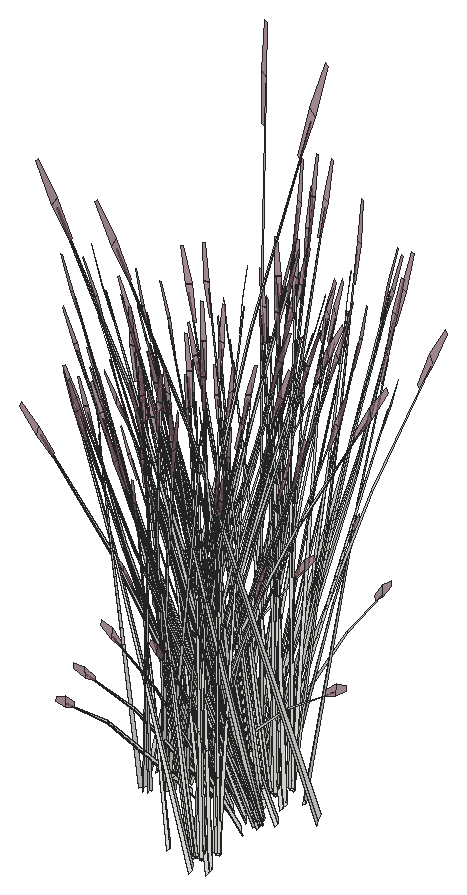
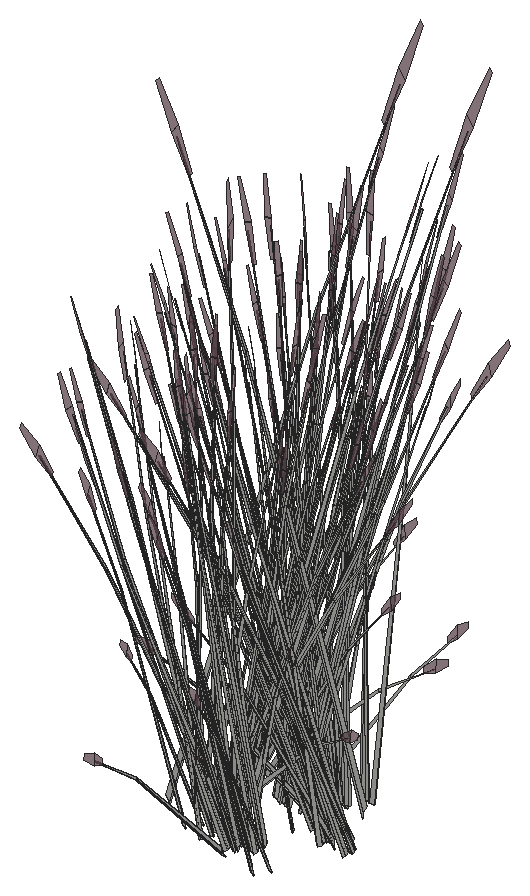
# SketchUp Ruby script. Lengths in inches.
U = 1.inch
M = Sketchup.active_model
def pt(a) = Geom::Point3d.new(a.map { |v| v * U })
def face(e, loops, mat)
  f = e.add_face(loops[0].map { |a| pt(a) })
  loops[1..].each { |l| e.add_face(l.map { |a| pt(a) }).erase! }
  f.material = f.back_material = mat if mat
  f
end
# faces: each face lists its corners as indices into pts; further lists are holes
def faces(e, pts, list, mat = nil) = list.each { |f| face(e, (f[0].is_a?(Array) ? f : [f]).map { |l| l.map { |i| pts[i] } }, mat) }
# xy, xz, yz: faces in a plane at the given z, y or x. An outline is a flat list of corners, or four numbers for a rectangle; further outlines are holes
def ring(l) = l.size == 4 ? [[l[0], l[1]], [l[2], l[1]], [l[2], l[3]], [l[0], l[3]]] : l.each_slice(2).to_a
def flat(e, list, mat, &to3) = list.each { |f| face(e, (f[0].is_a?(Array) ? f : [f]).map { |l| ring(l).map { |u, v| to3.(u, v) } }, mat) }
def xy(e, z, list, mat = nil) = flat(e, list, mat) { |x, y| [x, y, z] }
def xz(e, y, list, mat = nil) = flat(e, list, mat) { |x, z| [x, y, z] }
def yz(e, x, list, mat = nil) = flat(e, list, mat) { |y, z| [x, y, z] }
def lines(e, pts, list) = list.each { |a, b| e.add_line(pt(pts[a]), pt(pts[b])) }
# prism: a flat outline (further loops are holes) pulled along v
def prism(e, loops, v, mat = nil)
  f = face(e, loops, mat); d = Geom::Vector3d.new(v.map { |x| x * U })
  f.pushpull(f.normal.samedirection?(d) ? d.length : -d.length)
end
def box(e, o, s, mat = nil) = prism(e, [[o, [o[0] + s[0], o[1], o[2]], [o[0] + s[0], o[1] + s[1], o[2]], [o[0], o[1] + s[1], o[2]]]], [0, 0, s[2]], mat)
def at(x, y, z, deg = 0) = Geom::Transformation.translation(pt([x, y, z])) * Geom::Transformation.rotation(ORIGIN, Z_AXIS, deg.degrees)
def axes(o, x, y, z) = Geom::Transformation.new([*x, 0, *y, 0, *z, 0, *pt(o).to_a, 1])
def part(name) = M.definitions.add(name)
# library, detail: a bought-in or finely detailed component or shape, given as its bounding box
def library(name, o, s) = part(name).tap { |d| box(d.entities, o, s) }
def detail(e, o, s) = box(e.add_group.entities, o, s)
def put(e, d, t, mat = nil) = e.add_instance(d, t).tap { |i| i.material = mat if mat }
def group(e, t, mat = nil) = e.add_group.tap { |g| g.transformation = t; g.material = mat if mat }.entities
root = M.entities
M.materials.add("LightPink_Translucent").color = [144, 107, 117]
M.materials["LightPink_Translucent"].alpha = 0.75
c1 = part("blade")
p = [[2.15,0.21,22],[0,0.17,0],[0.09,0.45,0],[2.18,0.31,22],[2.29,0.31,22],[0.38,0.45,0],
  [2.48,0.24,33],[2.49,0.24,33],[2.48,0.22,33]]
faces(c1.entities,p,[[0,1,2,3],[4,5,2,3],[6,3,4,7],[8,0,3,6]])
c2 = part("seeds")
p = [[0.3,-0.1,1.38],[-0.01,-0.03,1.59],[-0.01,-0.03,0.03],[0.14,-0.07,-0.07],[0.29,-0.03,3],[0.15,0.01,3.11]]
faces(c2.entities,p,[[0,1,2,3],[1,0,4,5]],"LightPink_Translucent")
c3 = part("blade with seeds")
put(c3.entities,c1,at(0,0,0))
put(c3.entities,c2,axes([2.4,0.25,30.99],[1.5799,-0.05474,1.17369],[-0.12525,1.92788,0.29478],[-0.07173,-0.02425,1.56792]))
put(root,c3,axes([678.96,338.03,268.19],[0.10048,0.4599,0.29394],[-0.5744,0.12144,-0.37948],[-0.15428,-0.13179,0.72609]))
put(root,c3,axes([676.26,343.2,267.91],[0.07381,-0.03447,1.47228],[0.61004,0.22929,-0.13912],[-0.01434,0.19091,0.26054]))
put(root,c3,axes([674.61,339.19,268.13],[0.31051,0.46426,-0.58968],[-0.63919,0.25873,0.07116],[0.07261,0.22432,0.83415]))
put(root,c3,axes([682.41,338.67,267.22],[0.22574,-0.12077,1.42242],[0.19004,0.55807,0.11501],[-0.35439,0.12613,0.60807]))
put(root,c3,axes([680.14,341.15,266.76],[0.56221,0.23024,1.25546],[-0.55078,0.49601,0.49647],[-0.2467,-0.29398,1.05249]))
put(root,c3,axes([675.26,340.69,268.6875],[0.44958,-0.32756,-0.05385],[0.41194,0.35875,-0.24415],[0.029,0.10165,0.8053]))
put(root,c3,axes([678.12,341.81,268.43],[-0.01693,0.52814,-0.65454],[-0.71285,-0.03547,0.07899],[-0.07523,0.22375,0.92591]))
put(root,c3,axes([678.7,337.49,268.23],[0.72473,-0.14676,0.44623],[0.12578,0.57568,0.36794],[-0.17045,-0.16967,0.92337]))
put(root,c3,axes([683.71,338.09,266.77],[0.18493,-0.0826,1.46963],[0.06377,0.5767,0.11501],[-0.40056,0.07652,0.52526]))
put(root,c3,axes([674.85,339.29,267.89],[0.63954,0.14313,-0.42412],[-0.21921,0.49074,-0.32852],[0.05864,0.19758,0.81151]))
put(root,c3,axes([674.3,339.31,268.18],[0.63664,-0.26583,-0.10093],[0.31286,0.47181,-0.56021],[0.084,0.19882,0.85122]))
put(root,c3,axes([678.87,337.62,267.93],[0.29569,-0.36271,0.05337],[0.42107,0.21117,0.42015],[-0.13613,-0.11629,0.64067]))
put(root,c3,axes([677.88,342.55,266.79],[0.01429,-0.29475,1.28107],[0.64291,0.15569,0.17703],[-0.0557,0.31414,0.60492]))
put(root,c3,axes([681.72,338.47,267.91],[-0.10624,0.07413,1.45204],[0.00904,0.54162,-0.22964],[-0.24352,0.07044,0.11645]))
put(root,c3,axes([683.1,337.16,268.13],[-0.65035,-0.01375,-0.58968],[0.04368,-0.5789,0.07116],[-0.27552,-0.06109,0.83415]))
put(root,c3,axes([676.76,335.38,268.19],[-0.4402,0.30062,0.29394],[-0.41671,-0.34326,-0.37948],[0.0634,-0.1744,0.72609]))
put(root,c3,axes([679.51,336.54,267.91],[-0.09951,-0.08005,1.45204],[-0.66407,0.05075,-0.22964],[-0.10598,-0.19148,0.11645]))
put(root,c3,axes([682.06,338.16,267.76],[-0.54068,-0.15928,-0.29394],[0.1577,-0.46469,0.37948],[-0.21769,0.04261,0.72609]))
put(root,c3,axes([682.81,336.78,267.22],[0.24166,0.09837,1.42242],[-0.50011,0.41269,0.11501],[-0.3117,-0.18617,0.60807]))
put(root,c3,axes([678.27,341.99,268.15],[0.46573,0.38364,-0.47077],[-0.49199,0.33598,-0.36465],[-0.07086,0.19492,0.90078]))
put(root,c3,axes([678.06,341.7,268.19],[0.4402,-0.30062,0.29394],[0.41671,0.34326,-0.37948],[-0.0634,0.1744,0.72609]))
put(root,c3,axes([680.54,339.02,267.91],[0.08303,0.01531,1.47228],[0.25685,0.50448,-0.13912],[-0.16996,0.13241,0.26054]))
put(root,c3,axes([682.43,338.4,267.89],[-0.17625,0.51936,-0.42412],[-0.60429,-0.17802,-0.32852],[-0.2433,0.04762,0.81151]))
put(root,c3,axes([683.75,330.48,267.22],[0.22574,-0.12077,1.42242],[0.19004,0.55807,0.11501],[-0.35439,0.12613,0.60807]))
put(root,c3,axes([681.01,340.04,266.36],[-0.01777,-0.53759,1.17256],[0.80434,0.13935,0.49647],[-0.19024,0.29416,1.1068]))
put(root,c3,axes([682.89,337.28,267.89],[-0.47241,0.37822,-0.42412],[-0.41372,-0.39954,-0.32852],[-0.24002,-0.05755,0.81151]))
put(root,c3,axes([676.08,339.37,267.93],[-0.64708,0.13103,0.39842],[-0.1123,-0.514,0.32852],[0.15218,0.15149,0.82444]))
put(root,c3,axes([677.78,341.78,268.48],[0.71502,0.02829,-0.11203],[-0.01954,0.53563,-0.62183],[-0.04967,0.20629,0.94486]))
put(root,c3,axes([675.96,339.47,267.93],[-0.29569,0.36271,0.05337],[-0.42107,-0.21117,0.42015],[0.13613,0.11629,0.64067]))
put(root,c3,axes([675.21,338.27,267.22],[-0.14872,-0.18332,1.42242],[0.6872,-0.15433,0.11501],[0.15531,0.28779,0.60807]))
put(root,c3,axes([682.22,336.22,267.91],[0.04823,0.05698,1.47228],[-0.23252,0.51221,-0.13912],[-0.23548,0.00371,0.26054]))
put(root,c3,axes([680.52,337.77,268.18],[-0.63664,0.26583,-0.10093],[-0.31286,-0.47181,-0.56021],[-0.084,-0.19882,0.85122]))
put(root,c3,axes([679.97,337.8,267.89],[-0.63954,-0.14313,-0.42412],[0.21921,-0.49074,-0.32852],[-0.05864,-0.19758,0.81151]))
put(root,c3,axes([678.8,341.44,267.22],[-0.01592,-0.21915,1.42242],[0.69015,0.14538,0.11501],[-0.04269,0.3123,0.60807]))
put(root,c3,axes([682.76,335.88,267.91],[-0.13998,-0.00403,1.45204],[-0.44565,0.40302,-0.22964],[-0.23779,-0.08235,0.11645]))
put(root,c3,axes([682.18,338.11,267.93],[0.18381,-0.5206,0.39842],[0.60429,0.17802,0.32852],[-0.23764,0.03129,0.82444]))
put(root,c3,axes([682.4,337.96,268.18],[0.32734,0.51701,-0.10093],[-0.58097,0.25407,-0.56021],[-0.24483,0.06821,0.85122]))
put(root,c3,axes([683.14,336.88,268.18],[-0.03484,0.58066,-0.10093],[-0.65957,-0.01587,-0.56021],[-0.25402,-0.04034,0.85122]))
put(root,c3,axes([682.71,336.92,267.76],[-0.37017,-0.35748,-0.29394],[0.42268,-0.3384,0.37948],[-0.21476,-0.05149,0.72609]))
put(root,c3,axes([682.14,337.97,267.93],[-0.23895,-0.38931,0.05337],[0.43573,-0.19055,0.42015],[-0.19208,0.0376,0.64067]))
put(root,c3,axes([683.23,339.05,267.22],[0.1625,-0.17544,1.42242],[0.41029,0.47354,0.11501],[-0.28141,0.21565,0.60807]))
put(root,c3,axes([682.26,339.5,267.76],[-0.56631,0.0816,-0.29394],[-0.14954,-0.46647,0.37948],[-0.16229,0.12529,0.72609]))
put(root,c3,axes([680.21,337.89,268.13],[-0.31051,-0.46426,-0.58968],[0.63919,-0.25873,0.07116],[-0.07261,-0.22432,0.83415]))
put(root,c3,axes([675.86,339.05,268.19],[-0.10048,-0.4599,0.29394],[0.5744,-0.12144,-0.37948],[0.15428,0.13179,0.72609]))
put(root,c3,axes([676.25,336.41,267.71],[-0.56218,-0.29666,1.14775],[0.59361,-0.46189,0.49522],[0.18138,0.27836,1.10941]))
put(root,c3,axes([682.33,339.4,267.93],[-0.16135,-0.52549,0.39842],[0.63294,-0.0912,0.32852],[-0.18654,0.12359,0.82444]))
put(root,c3,axes([675.31,339.7,267.91],[0.00193,-0.06913,1.47228],[0.55753,-0.30498,-0.13912],[0.19366,0.10886,0.26054]))
put(root,c3,axes([677.16,335.11,267.93],[0.53464,0.0266,0.05337],[-0.01466,0.40172,0.42015],[0.05594,-0.15388,0.64067]))
put(root,c3,axes([682.66,336.79,268.23],[0.53728,-0.42137,0.44623],[0.46337,0.44748,0.36794],[-0.25207,-0.07773,0.92337]))
put(root,c3,axes([681.875,330.83,267.91],[0.08303,0.01531,1.47228],[0.25685,0.50448,-0.13912],[-0.16996,0.13241,0.26054]))
put(root,c3,axes([680.33,337.96,268.19],[-0.19614,0.43908,0.29394],[-0.57222,-0.12807,-0.37948],[-0.05247,-0.17678,0.72609]))
put(root,c3,axes([682.21,339.3,267.93],[-0.44663,-0.24013,0.05337],[0.26003,-0.34195,0.42015],[-0.14319,0.11055,0.64067]))
put(root,c3,axes([679.28,342.56,268.2],[-0.64106,-0.14927,0.44225],[0.21921,-0.49074,0.36465],[0.03852,0.19299,0.91512]))
put(root,c3,axes([676.99,335.07,267.93],[0.46327,0.38957,0.39842],[-0.49199,0.33598,0.32852],[0.08546,-0.18277,0.82444]))
put(root,c3,axes([679.11,342.59,267.93],[-0.47939,0.19405,0.05337],[-0.23464,-0.35385,0.42015],[0.0463,0.15598,0.64067]))
put(root,c3,axes([683.11,339.48,267.22],[0.12114,-0.19625,1.42242],[0.50818,0.40613,0.11501],[-0.22925,0.25313,0.60807]))
put(root,c3,axes([682.63,338.11,268.19],[0.54068,0.15928,0.29394],[-0.1577,0.46469,-0.37948],[-0.21769,0.04261,0.72609]))
put(root,c3,axes([682.72,339.56,267.89],[0.16713,0.52135,-0.42412],[-0.63294,0.0912,-0.32852],[-0.18138,0.14003,0.81151]))
put(root,c3,axes([677.53,336.3125,268.19],[-0.56631,0.0816,0.29394],[-0.14954,-0.46647,-0.37948],[0.16229,-0.12529,0.72609]))
put(root,c3,axes([682.9,336.79,267.93],[0.03276,-0.43418,0.05337],[0.49468,0.0119,0.42015],[-0.18949,-0.04543,0.64067]))
put(root,c3,axes([681.74,340.5,267.91],[-0.01617,0.11299,1.45204],[0.45894,0.39307,-0.22964],[-0.12015,0.18588,0.11645]))
put(root,c3,axes([684.42,336.04,268.51],[-0.4342,0.54737,-0.11304],[-0.6288,-0.31535,-0.62743],[-0.21858,-0.15465,0.95337]))
put(root,c3,axes([680.27,337.5,267.76],[0.19614,-0.43908,-0.29394],[0.57222,0.12807,0.37948],[-0.05247,-0.17678,0.72609]))
put(root,c3,axes([683.24,337.11,268.19],[0.37017,0.35748,0.29394],[-0.42268,0.3384,-0.37948],[-0.21476,-0.05149,0.72609]))
put(root,c3,axes([684.57,330.86,267.22],[0.1625,-0.17544,1.42242],[0.41029,0.47354,0.11501],[-0.28141,0.21565,0.60807]))
put(root,c3,axes([683.6,331.32,267.76],[-0.56631,0.0816,-0.29394],[-0.14954,-0.46647,0.37948],[-0.16229,0.12529,0.72609]))
put(root,c3,axes([684.23,336.48,268.13],[-0.55475,-0.27598,-0.58968],[0.39425,-0.48361,0.07116],[-0.20099,-0.16478,0.83415]))
put(root,c3,axes([683.98,336.49,267.89],[-0.64198,0.13573,-0.42412],[-0.1123,-0.514,-0.32852],[-0.17243,-0.1473,0.81151]))
put(root,c3,axes([679.36,342.66,267.76],[-0.19614,0.43908,-0.29394],[-0.57222,-0.12807,0.37948],[0.05247,0.17678,0.72609]))
put(root,c3,axes([675.8125,339.29,268.18],[0.38768,-0.48872,-0.10093],[0.56143,0.28156,-0.56021],[0.19516,0.13808,0.85122]))
put(root,c3,axes([677.82,336.36,268.18],[-0.60181,-0.31483,-0.10093],[0.34671,-0.45593,-0.56021],[0.17003,-0.15849,0.85122]))
put(root,c3,axes([682.43,339.1875,268.18],[0.60181,0.31483,-0.10093],[-0.34671,0.45593,-0.56021],[-0.17003,0.15849,0.85122]))
put(root,c3,axes([683.67,331.22,267.93],[-0.16135,-0.52549,0.39842],[0.63294,-0.0912,0.32852],[-0.18654,0.12359,0.82444]))
put(root,c3,axes([676.27,339.05,267.89],[0.64198,-0.13573,-0.42412],[0.1123,0.514,-0.32852],[0.17243,0.1473,0.81151]))
put(root,c3,axes([683.54,331.11,267.93],[-0.44663,-0.24013,0.05337],[0.26003,-0.34195,0.42015],[-0.14319,0.11055,0.64067]))
put(root,c3,axes([680.51,337.5625,267.93],[0.47939,-0.19405,0.05337],[0.23464,0.35385,0.42015],[-0.0463,-0.15598,0.64067]))
put(root,c3,axes([678.95,343.4375,267.91],[0.08247,0.09194,1.45204],[0.66552,0.03612,-0.22964],[0.06692,0.20277,0.11645]))
put(root,c3,axes([677.01,338.43,268.19],[-0.37017,-0.35748,0.29394],[0.42268,-0.3384,-0.37948],[0.21476,0.05149,0.72609]))
put(root,c3,axes([680.34,337.6,267.93],[0.64106,0.14927,0.39842],[-0.21921,0.49074,0.32852],[-0.03852,-0.19299,0.82444]))
put(root,c3,axes([681.43,340.55,268.6875],[0.5741,0.15241,-0.05385],[-0.1766,0.46909,-0.24415],[-0.0939,0.07122,0.8053]))
put(root,c3,axes([684.45,331.29,267.22],[0.12114,-0.19625,1.42242],[0.50818,0.40613,0.11501],[-0.22925,0.25313,0.60807]))
put(root,c3,axes([677.34,338.76,267.93],[-0.03276,0.43418,0.05337],[-0.49468,-0.0119,0.42015],[0.18949,0.04543,0.64067]))
put(root,c3,axes([682.72,339.23,268.19],[0.56631,-0.0816,0.29394],[0.14954,0.46647,-0.37948],[-0.16229,0.12529,0.72609]))
put(root,c3,axes([679.29,342.2,268.19],[0.19614,-0.43908,0.29394],[0.57222,0.12807,-0.37948],[0.05247,0.17678,0.72609]))
put(root,c3,axes([677.39,338.62,267.93],[-0.47971,0.37622,0.39842],[-0.41372,-0.39954,0.32852],[0.22506,0.0694,0.82444]))
put(root,c3,axes([677.52,335.98,267.89],[-0.16713,-0.52135,-0.42412],[0.63294,-0.0912,-0.32852],[0.18138,-0.14003,0.81151]))
put(root,c3,axes([678.64,338.67,267.26],[-0.12452,-0.47997,-0.02898],[0.58854,-0.11034,-0.1314],[0.1229,0.03043,0.43341]))
put(root,c3,axes([677.62,337.43,268.19],[-0.54068,-0.15928,0.29394],[0.1577,-0.46469,-0.37948],[0.21769,-0.04261,0.72609]))
put(root,c3,axes([684.0625,331.37,267.89],[0.16713,0.52135,-0.42412],[-0.63294,0.0912,-0.32852],[-0.18138,0.14003,0.81151]))
put(root,c3,axes([684.26,334.73,267.91],[-0.01214,0.06844,1.47228],[-0.59861,0.24837,-0.13912],[-0.17615,-0.12696,0.26054]))
put(root,c3,axes([683.07,332.31,267.91],[-0.01617,0.11299,1.45204],[0.45894,0.39307,-0.22964],[-0.12015,0.18588,0.11645]))
put(root,c3,axes([679.41,342.26,268.13],[0.31051,0.46426,-0.58968],[-0.63919,0.25873,0.07116],[0.07261,0.22432,0.83415]))
put(root,c3,axes([683.25,340.47,267.93],[-0.46327,-0.38957,0.39842],[0.49199,-0.33598,0.32852],[-0.08546,0.18277,0.82444]))
put(root,c3,axes([684.04,336.12,267.76],[-0.10048,-0.4599,-0.29394],[0.5744,-0.12144,0.37948],[-0.15428,-0.13179,0.72609]))
put(root,c3,axes([678.04,336.24,267.93],[0.44663,0.24013,0.05337],[-0.26003,0.34195,0.42015],[0.14319,-0.11055,0.64067]))
put(root,c3,axes([683.08,340.43,267.93],[-0.53464,-0.0266,0.05337],[0.01466,-0.40172,0.42015],[-0.05594,0.15388,0.64067]))
put(root,c3,axes([680.0625,343.76,268.6875],[0.44958,-0.32756,-0.05385],[0.41194,0.35875,-0.24415],[0.029,0.10165,0.8053]))
put(root,c3,axes([683.25,340.58,267.76],[-0.4402,0.30062,-0.29394],[-0.41671,-0.34326,0.37948],[-0.0634,0.1744,0.72609]))
put(root,c3,axes([677.92,336.14,267.93],[0.16135,0.52549,0.39842],[-0.63294,0.0912,0.32852],[0.18654,-0.12359,0.82444]))
put(root,c3,axes([683.76,331,268.18],[0.60181,0.31483,-0.10093],[-0.34671,0.45593,-0.56021],[-0.17003,0.15849,0.85122]))
put(root,c3,axes([679.65,342.36,267.89],[0.63954,0.14313,-0.42412],[-0.21921,0.49074,-0.32852],[0.05864,0.19758,0.81151]))
put(root,c3,axes([676.2,337.7,267.22],[-0.24166,-0.09837,1.42242],[0.50011,-0.41269,0.11501],[0.3117,0.18617,0.60807]))
put(root,c3,axes([679.1,342.38,268.18],[0.63664,-0.26583,-0.10093],[0.31286,0.47181,-0.56021],[0.084,0.19882,0.85122]))
put(root,c3,axes([684.38,336.49,268.19],[0.10048,0.4599,0.29394],[-0.5744,0.12144,-0.37948],[-0.15428,-0.13179,0.72609]))
put(root,c3,axes([681.68,341.65,267.91],[0.07381,-0.03447,1.47228],[0.61004,0.22929,-0.13912],[-0.01434,0.19091,0.26054]))
put(root,c3,axes([679.3,336.22,267.91],[-0.08498,-0.00434,1.47228],[-0.35287,-0.46464,-0.13912],[0.14171,-0.15278,0.26054]))
put(root,c3,axes([682.35,337.11,267.91],[-0.06607,0.04361,1.47228],[-0.64734,-0.14714,-0.13912],[-0.02343,-0.19032,0.26054]))
put(root,c3,axes([681.84,338.37,268.18],[-0.71502,-0.02829,-0.10093],[0.01954,-0.53563,-0.56021],[0.04967,-0.20629,0.85122]))
put(root,c3,axes([677.99,336.04,267.76],[0.56631,-0.0816,-0.29394],[0.14954,0.46647,0.37948],[0.16229,-0.12529,0.72609]))
put(root,c3,axes([685.5625,339.6,266.76],[0.56221,0.23024,1.25546],[-0.55078,0.49601,0.49647],[-0.2467,-0.29398,1.05249]))
put(root,c3,axes([677.54,336.19,268.13],[0.33983,-0.45051,-0.58968],[0.59551,0.32017,0.07116],[0.20291,-0.16322,0.83415]))
put(root,c3,axes([678.11,337.57,267.93],[0.23895,0.38931,0.05337],[-0.43573,0.19055,0.42015],[0.19208,-0.0376,0.64067]))
put(root,c3,axes([682.77,332.37,268.6875],[0.5741,0.15241,-0.05385],[-0.1766,0.46909,-0.24415],[-0.0939,0.07122,0.8053]))
put(root,c3,axes([677.53,338.62,267.76],[0.37017,0.35748,-0.29394],[-0.42268,0.3384,0.37948],[0.21476,0.05149,0.72609]))
put(root,c3,axes([677.11,338.66,268.18],[0.03484,-0.58066,-0.10093],[0.65957,0.01587,-0.56021],[0.25402,0.04034,0.85122]))
put(root,c3,axes([677.85,337.58,268.18],[-0.32734,-0.51701,-0.10093],[0.58097,-0.25407,-0.56021],[0.24483,-0.06821,0.85122]))
put(root,c3,axes([684.06,331.04,268.19],[0.56631,-0.0816,0.29394],[0.14954,0.46647,-0.37948],[-0.16229,0.12529,0.72609]))
put(root,c3,axes([678.0625,337.43,267.93],[-0.18381,0.5206,0.39842],[-0.60429,-0.17802,0.32852],[0.23764,-0.03129,0.82444]))
put(root,c3,axes([681.5625,338.45,268.19],[-0.4402,0.30062,0.29394],[-0.41671,-0.34326,-0.37948],[0.0634,-0.1744,0.72609]))
put(root,c3,axes([683.55,340.27,268.43],[-0.01693,0.52814,-0.65454],[-0.71285,-0.03547,0.07899],[-0.07523,0.22375,0.92591]))
put(root,c3,axes([681.36,338.17,267.89],[-0.46573,-0.38364,-0.42412],[0.49199,-0.33598,-0.32852],[0.07086,-0.19492,0.81151]))
put(root,c3,axes([684.125,335.95,268.23],[0.72473,-0.14676,0.44623],[0.12578,0.57568,0.36794],[-0.17045,-0.16967,0.92337]))
put(root,c3,axes([684.29,336.07,267.93],[0.29569,-0.36271,0.05337],[0.42107,0.21117,0.42015],[-0.13613,-0.11629,0.64067]))
put(root,c3,axes([683.31,341.01,266.79],[0.01429,-0.29475,1.28107],[0.64291,0.15569,0.17703],[-0.0557,0.31414,0.60492]))
put(root,c3,axes([677.68,338.31,267.91],[0.13956,-0.00966,1.45204],[0.38281,-0.44358,-0.22964],[0.24825,0.05855,0.11645]))
put(root,c3,axes([684.59,332.28,267.93],[-0.46327,-0.38957,0.39842],[0.49199,-0.33598,0.32852],[-0.08546,0.18277,0.82444]))
put(root,c3,axes([677.82,337.14,267.89],[0.17625,-0.51936,-0.42412],[0.60429,0.17802,-0.32852],[0.2433,-0.04762,0.81151]))
put(root,c3,axes([684.42,332.24,267.93],[-0.53464,-0.0266,0.05337],[0.01466,-0.40172,0.42015],[-0.05594,0.15388,0.64067]))
put(root,c3,axes([680.88,342.4375,267.93],[-0.64708,0.13103,0.39842],[-0.1123,-0.514,0.32852],[0.15218,0.15149,0.82444]))
put(root,c3,axes([680.76,342.54,267.93],[-0.29569,0.36271,0.05337],[-0.42107,-0.21117,0.42015],[0.13613,0.11629,0.64067]))
put(root,c3,axes([684.59,332.4,267.76],[-0.4402,0.30062,-0.29394],[-0.41671,-0.34326,0.37948],[-0.0634,0.1744,0.72609]))
put(root,c3,axes([680.01,341.34,267.22],[-0.14872,-0.18332,1.42242],[0.6872,-0.15433,0.11501],[0.15531,0.28779,0.60807]))
put(root,c3,axes([678.1875,337.38,267.76],[0.54068,0.15928,-0.29394],[-0.1577,0.46469,0.37948],[0.21769,-0.04261,0.72609]))
